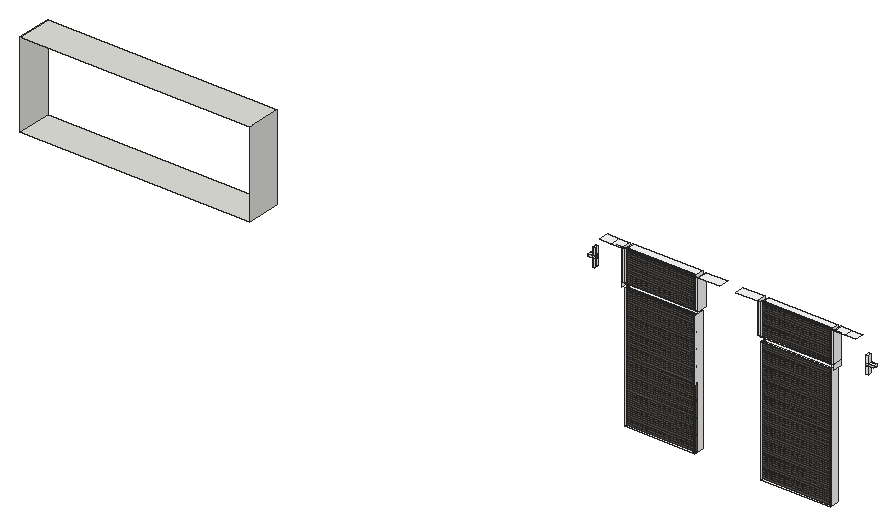
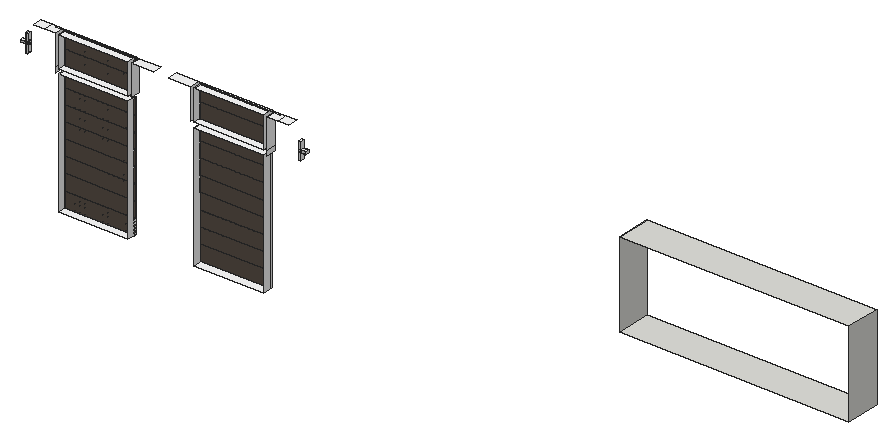
# SketchUp Ruby script. Lengths in inches.
U = 1.inch
M = Sketchup.active_model
def pt(a) = Geom::Point3d.new(a.map { |v| v * U })
def face(e, loops, mat)
  f = e.add_face(loops[0].map { |a| pt(a) })
  loops[1..].each { |l| e.add_face(l.map { |a| pt(a) }).erase! }
  f.material = f.back_material = mat if mat
  f
end
# faces: each face lists its corners as indices into pts; further lists are holes
def faces(e, pts, list, mat = nil) = list.each { |f| face(e, (f[0].is_a?(Array) ? f : [f]).map { |l| l.map { |i| pts[i] } }, mat) }
# xy, xz, yz: faces in a plane at the given z, y or x. An outline is a flat list of corners, or four numbers for a rectangle; further outlines are holes
def ring(l) = l.size == 4 ? [[l[0], l[1]], [l[2], l[1]], [l[2], l[3]], [l[0], l[3]]] : l.each_slice(2).to_a
def flat(e, list, mat, &to3) = list.each { |f| face(e, (f[0].is_a?(Array) ? f : [f]).map { |l| ring(l).map { |u, v| to3.(u, v) } }, mat) }
def xy(e, z, list, mat = nil) = flat(e, list, mat) { |x, y| [x, y, z] }
def xz(e, y, list, mat = nil) = flat(e, list, mat) { |x, z| [x, y, z] }
def yz(e, x, list, mat = nil) = flat(e, list, mat) { |y, z| [x, y, z] }
def lines(e, pts, list) = list.each { |a, b| e.add_line(pt(pts[a]), pt(pts[b])) }
# prism: a flat outline (further loops are holes) pulled along v
def prism(e, loops, v, mat = nil)
  f = face(e, loops, mat); d = Geom::Vector3d.new(v.map { |x| x * U })
  f.pushpull(f.normal.samedirection?(d) ? d.length : -d.length)
end
def box(e, o, s, mat = nil) = prism(e, [[o, [o[0] + s[0], o[1], o[2]], [o[0] + s[0], o[1] + s[1], o[2]], [o[0], o[1] + s[1], o[2]]]], [0, 0, s[2]], mat)
def at(x, y, z, deg = 0) = Geom::Transformation.translation(pt([x, y, z])) * Geom::Transformation.rotation(ORIGIN, Z_AXIS, deg.degrees)
def axes(o, x, y, z) = Geom::Transformation.new([*x, 0, *y, 0, *z, 0, *pt(o).to_a, 1])
def part(name) = M.definitions.add(name)
# library, detail: a bought-in or finely detailed component or shape, given as its bounding box
def library(name, o, s) = part(name).tap { |d| box(d.entities, o, s) }
def detail(e, o, s) = box(e.add_group.entities, o, s)
def put(e, d, t, mat = nil) = e.add_instance(d, t).tap { |i| i.material = mat if mat }
def group(e, t, mat = nil) = e.add_group.tap { |g| g.transformation = t; g.material = mat if mat }.entities
root = M.entities
M.materials.add("[Color_000]").color = [255, 255, 255]
M.materials.add("[Color_C20]").color = [102, 91, 81]
c1 = part("Gate slat")
xy(c1.entities,0,[[0.39,114.16,6.3,114.17]])
xy(c1.entities,0,[[0.39,0,6.3,114.16]],"[Color_C20]")
xy(c1.entities,0.39,[[0.39,0,0.79,114.17],[0.98,0,2.07,114.17],[2.36,0,3.2,114.17],[3.59,0,4.37,114.17],[4.56,0,5.71,114.17],
  [5.91,0,6.3,114.17]],"[Color_C20]")
xy(c1.entities,0.79,[[0.39,0,0.79,114.17],[0.98,0,2.07,114.17],[2.36,0,3.2,114.17],[3.59,0,4.37,114.17],[4.56,0,5.71,114.17],
  [5.91,0,6.3,114.17]],"[Color_C20]")
xy(c1.entities,0.99,[[1.13,0,1.21,114.16],[1.87,0,1.94,114.16],[2.61,0,2.68,114.16],[3.35,0,3.42,114.16],[4.08,0,4.16,114.16],
  [4.82,0,4.9,114.16],[5.5625,0,5.63,114.16],[6.3,0,6.37,114.16]],"[Color_C20]")
xy(c1.entities,1.18,[[0.39,114.16,3.35,114.17],[3.35,114.16,6.3,114.17]])
xy(c1.entities,1.18,[[0.39,0,1.13,114.16],[1.21,0,1.87,114.16],[1.94,0,2.61,114.16],[2.68,0,3.35,114.16],[3.42,0,4.08,114.16],
  [4.16,0,4.82,114.16],[4.9,0,5.5625,114.16],[5.63,0,6.3,114.16]],"[Color_C20]")
xz(c1.entities,0,[[[0.39,0,6.3,0,6.3,0.39,5.91,0.39,5.91,0.79,6.3,0.79,6.3,1.18,5.63,1.18,5.63,0.99,5.5625,0.99,5.5625,1.18,4.9,1.18,4.9,0.99,4.82,0.99,4.82,1.18,4.16,1.18,4.16,0.99,4.08,0.99,4.08,1.18,3.42,1.18,3.42,0.99,3.35,0.99,3.35,1.18,2.68,1.18,2.68,0.99,2.61,0.99,2.61,1.18,1.94,1.18,1.94,0.99,1.87,0.99,1.87,1.18,1.21,1.18,1.21,0.99,1.13,0.99,1.13,1.18,0.39,1.18,0.39,0.79,0.79,0.79,0.79,0.39,0.39,0.39],[4.56,0.39,5.71,0.79],[0.98,0.39,2.07,0.79],[2.36,0.39,3.2,0.79],[3.59,0.39,4.37,0.79]],[6.3,0.99,6.37,1.18]],"[Color_C20]")
xz(c1.entities,114.16,[[1.13,0.99,1.21,1.18],[1.87,0.99,1.94,1.18],[2.61,0.99,2.68,1.18],[3.35,0.99,3.42,1.18],[4.08,0.99,4.16,1.18],
  [4.82,0.99,4.9,1.18],[5.5625,0.99,5.63,1.18]],"[Color_C20]")
xz(c1.entities,114.17,[[[0.39,0,0.39,0.39,0.79,0.39,0.79,0.79,0.39,0.79,0.39,1.18,6.3,1.18,6.3,0.79,5.91,0.79,5.91,0.39,6.3,0.39,6.3,0],[4.56,0.39,5.71,0.79],[0.98,0.39,2.07,0.79],[2.36,0.39,3.2,0.79],[3.59,0.39,4.37,0.79]]],"[Color_C20]")
yz(c1.entities,0.39,[[114.16,0,114.17,0.39],[114.16,0.79,114.17,1.18]])
yz(c1.entities,0.39,[[0,0,114.16,0.39],[0,0.79,114.16,1.18]],"[Color_C20]")
yz(c1.entities,0.79,[[0,0.39,114.17,0.79]],"[Color_C20]")
yz(c1.entities,0.98,[[0,0.39,114.17,0.79]],"[Color_C20]")
yz(c1.entities,1.13,[[0,0.99,114.16,1.18]],"[Color_C20]")
yz(c1.entities,1.21,[[0,0.99,114.16,1.18]],"[Color_C20]")
yz(c1.entities,1.87,[[0,0.99,114.16,1.18]],"[Color_C20]")
yz(c1.entities,1.94,[[0,0.99,114.16,1.18]],"[Color_C20]")
yz(c1.entities,2.07,[[0,0.39,114.17,0.79]],"[Color_C20]")
yz(c1.entities,2.36,[[0,0.39,114.17,0.79]],"[Color_C20]")
yz(c1.entities,2.61,[[0,0.99,114.16,1.18]],"[Color_C20]")
yz(c1.entities,2.68,[[0,0.99,114.16,1.18]],"[Color_C20]")
yz(c1.entities,3.2,[[0,0.39,114.17,0.79]],"[Color_C20]")
yz(c1.entities,3.35,[[0,0.99,114.16,1.18]],"[Color_C20]")
yz(c1.entities,3.42,[[0,0.99,114.16,1.18]],"[Color_C20]")
yz(c1.entities,3.59,[[0,0.39,114.17,0.79]],"[Color_C20]")
yz(c1.entities,4.08,[[0,0.99,114.16,1.18]],"[Color_C20]")
yz(c1.entities,4.16,[[0,0.99,114.16,1.18]],"[Color_C20]")
yz(c1.entities,4.37,[[0,0.39,114.17,0.79]],"[Color_C20]")
yz(c1.entities,4.56,[[0,0.39,114.17,0.79]],"[Color_C20]")
yz(c1.entities,4.82,[[0,0.99,114.16,1.18]],"[Color_C20]")
yz(c1.entities,4.9,[[0,0.99,114.16,1.18]],"[Color_C20]")
yz(c1.entities,5.5625,[[0,0.99,114.16,1.18]],"[Color_C20]")
yz(c1.entities,5.63,[[0,0.99,114.16,1.18]],"[Color_C20]")
yz(c1.entities,5.71,[[0,0.39,114.17,0.79]],"[Color_C20]")
yz(c1.entities,5.91,[[0,0.39,114.17,0.79]],"[Color_C20]")
yz(c1.entities,6.3,[[114.16,0,114.17,0.39],[114.16,0.79,114.17,1.18]])
yz(c1.entities,6.3,[[0,0,114.16,0.39],[0,0.79,114.16,0.99],[0,0.99,114.16,1.18]],"[Color_C20]")
yz(c1.entities,6.37,[[0,0.99,114.16,1.18]],"[Color_C20]")
p = [[0,0,0],[0.39,0,0]]
lines(c1.entities,p,[[0,1]])
c2 = part("Vertical gate panel")
put(c2.entities,c1,axes([0,1.18,0],[3.67755,0,0],[0,0,2.40086],[0,-1,0]))
put(c2.entities,c1,axes([21.72,1.18,0],[3.67755,0,0],[0,0,2.40086],[0,-1,0]))
xy(root,22.97,[[321.64,182.1,352.12,186.51],[381.28,182.1,411.76,186.22]],"[Color_000]")
xy(root,57.77,[[69.92,165,170.46,180]])
xy(root,77.25,[[321.64,182.1,352.12,186.51],[381.28,182.1,411.76,186.22]],"[Color_000]")
xy(root,79.29,[[321.64,182.1,352.12,186.51],[381.28,182.1,411.76,186.22]],"[Color_000]")
xy(root,79.68,[[426.21,183.55,427.3,185.11],[306.1,183.66,307.1875,185.32]],"[Color_000]")
xy(root,82.91,[[426.21,183.55,427.3,185.11],[306.1,183.66,307.1875,185.32]],"[Color_000]")
xy(root,83.06,[[426.21,183.55,427.3,185.11],[427.3,183.55,429.53,185.11],[303.875,183.66,306.1,185.32],[306.1,183.66,307.1875,185.32]],"[Color_000]")
xy(root,84.04,[[426.21,183.55,427.3,185.11],[427.3,183.55,429.53,185.11],[303.875,183.66,306.1,185.32],[306.1,183.66,307.1875,185.32]],"[Color_000]")
xy(root,84.2,[[426.21,183.55,427.3,185.11],[306.1,183.66,307.1875,185.32]],"[Color_000]")
xy(root,87.3125,[[426.21,183.55,427.3,185.11],[306.1,183.66,307.1875,185.32]],"[Color_000]")
xy(root,92.71,[[310.6,182.1,315.39,186.51],[315.39,182.1,320.1875,186.51],[321.64,182.1,352.12,186.51],[353.58,182.1,363.16,186.51],[370.24,182.1,379.83,186.22],
  [381.28,182.1,411.76,186.22],[413.21,182.1,418.01,186.22],[418.01,182.1,422.8,186.22]],"[Color_000]")
xy(root,95.29,[[69.92,165,170.46,180]])
xz(root,182.1,[[320.1875,79.29,321.64,92.71],[352.12,79.29,353.58,92.71],[379.83,79.29,381.28,92.71],[411.76,79.29,413.21,92.71]],"[Color_000]")
xz(root,183.55,[[426.21,79.68,427.3,82.91],[426.21,83.06,429.53,84.04],[426.21,84.2,427.3,87.3125]],"[Color_000]")
xz(root,183.66,[[306.1,79.68,307.1875,82.91],[303.875,83.06,307.1875,84.04],[306.1,84.2,307.1875,87.3125]],"[Color_000]")
xz(root,185.11,[[426.21,79.68,427.3,82.91],[426.21,83.06,427.3,83.44],[427.3,83.06,427.3,83.44,426.21,83.44,426.21,84.04,429.53,84.04,429.53,83.06],[426.21,84.2,427.3,87.3125]],"[Color_000]")
xz(root,185.32,[[306.1,79.68,307.1875,82.91],[303.875,83.06,303.875,84.04,307.1875,84.04,307.1875,83.44,306.1,83.44,306.1,83.06],[306.1,83.06,307.1875,83.44],[306.1,84.2,307.1875,87.3125]],"[Color_000]")
yz(root,69.92,[[165,57.77,180,95.29]])
yz(root,170.46,[[165,57.77,180,95.29]])
yz(root,303.875,[[183.66,83.06,185.32,84.04]],"[Color_000]")
yz(root,306.1,[[183.66,79.68,185.32,82.91],[183.66,84.2,185.32,87.3125]],"[Color_000]")
yz(root,320.1875,[[182.1,77.25,186.51,79.29],[182.1,79.29,186.51,92.71]],"[Color_000]")
yz(root,321.64,[[182.1,22.97,186.51,77.25],[182.1,79.29,186.51,92.71]],"[Color_000]")
yz(root,352.12,[[182.1,22.97,186.51,77.25],[182.1,79.29,186.51,92.71]],"[Color_000]")
yz(root,353.58,[[182.1,79.29,186.51,92.71]],"[Color_000]")
yz(root,379.83,[[182.1,79.29,186.22,92.71]],"[Color_000]")
yz(root,381.28,[[182.1,22.97,186.22,77.25],[182.1,79.29,186.22,92.71]],"[Color_000]")
yz(root,411.76,[[182.1,22.97,186.22,77.25],[182.1,79.29,186.22,92.71]],"[Color_000]")
yz(root,413.21,[[182.1,77.25,186.22,79.29],[182.1,79.29,186.22,92.71]],"[Color_000]")
yz(root,427.3,[[183.55,79.68,185.11,82.91],[183.55,84.2,185.11,87.3125]],"[Color_000]")
p = [[416.23,182.78,92.7],[381.28,182.78,92.7],[411.76,182.78,79.79],[411.76,182.78,22.97],[317.17,182.83,92.7],[352.12,182.83,92.7],
  [321.65,182.83,79.79],[321.65,182.83,22.97],[307.1875,185.32,83.06],[307.1875,185.32,82.91]]
lines(root,p,[[0,1],[2,3],[4,5],[6,7],[8,9]])
put(root,c2,axes([381.28,182.78,22.8],[0,0,0.3108],[0,0.27902,0],[0.11119,0,0]))
put(root,c2,axes([352.125,182.83,22.8],[0,0,0.3108],[0,0.299,0],[-0.11119,0,0]))
put(root,c2,axes([381.28,182.78,36.3],[0,0,0.3108],[0,0.27902,0],[0.11119,0,0]))
put(root,c2,axes([352.125,182.83,36.3],[0,0,0.3108],[0,0.299,0],[-0.11119,0,0]))
put(root,c2,axes([381.28,182.78,49.8],[0,0,0.3108],[0,0.27902,0],[0.11119,0,0]))
put(root,c2,axes([352.12,182.83,49.8],[0,0,0.3108],[0,0.299,0],[-0.11119,0,0]))
put(root,c2,axes([381.28,182.78,63.3],[0,0,0.3108],[0,0.27902,0],[0.11119,0,0]))
put(root,c2,axes([352.12,182.83,63.3],[0,0,0.3108],[0,0.299,0],[-0.11119,0,0]))
put(root,c2,axes([381.28,182.78,78.47],[0,0,0.31699],[0,0.27902,0],[0.11119,0,0]))
put(root,c2,axes([352.12,182.83,78.47],[0,0,0.31699],[0,0.299,0],[-0.11119,0,0]))
